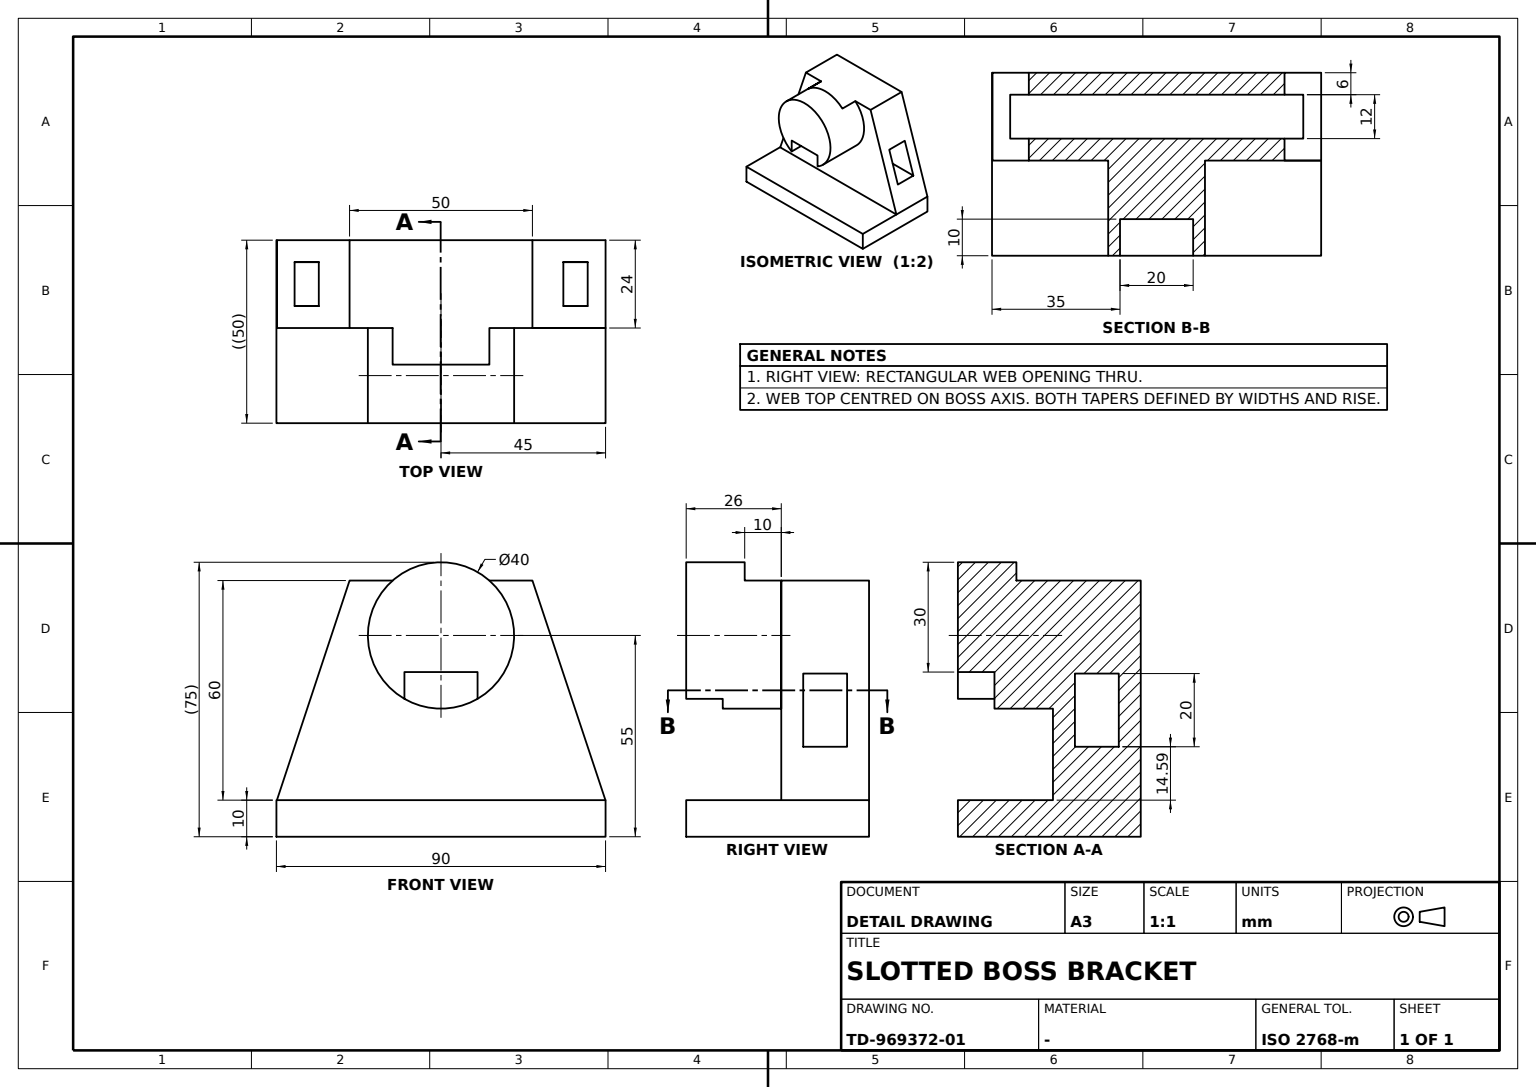
ISO-10303-21;
HEADER;
FILE_DESCRIPTION((''),'2;1');
FILE_NAME('','',(''),(''),'','','');
FILE_SCHEMA(('AUTOMOTIVE_DESIGN'));
ENDSEC;
DATA;
#1=APPLICATION_CONTEXT('');
#2=PRODUCT_CONTEXT('',#1,'mechanical');
#3=PRODUCT('','','',(#2));
#4=PRODUCT_DEFINITION_FORMATION('','',#3);
#5=PRODUCT_DEFINITION_CONTEXT('',#1,'design');
#6=PRODUCT_DEFINITION('','',#4,#5);
#7=PRODUCT_DEFINITION_SHAPE('','',#6);
#8=(LENGTH_UNIT()NAMED_UNIT(*)SI_UNIT(.MILLI.,.METRE.));
#9=(NAMED_UNIT(*)PLANE_ANGLE_UNIT()SI_UNIT($,.RADIAN.));
#10=(NAMED_UNIT(*)SI_UNIT($,.STERADIAN.)SOLID_ANGLE_UNIT());
#11=UNCERTAINTY_MEASURE_WITH_UNIT(LENGTH_MEASURE(0.005),#8,'distance_accuracy_value','');
#12=(GEOMETRIC_REPRESENTATION_CONTEXT(3)GLOBAL_UNCERTAINTY_ASSIGNED_CONTEXT((#11))GLOBAL_UNIT_ASSIGNED_CONTEXT((#8,#9,#10))REPRESENTATION_CONTEXT('',''));
#13=CARTESIAN_POINT('',(89.863327,0.,10.));
#14=VERTEX_POINT('',#13);
#15=CARTESIAN_POINT('',(90.,0.,10.));
#16=VERTEX_POINT('',#15);
#17=CARTESIAN_POINT('',(0.,0.,10.));
#18=DIRECTION('',(1.,0.,0.));
#19=VECTOR('',#18,1000.);
#20=LINE('',#17,#19);
#21=EDGE_CURVE('',#14,#16,#20,.T.);
#22=ORIENTED_EDGE('',*,*,#21,.F.);
#23=CARTESIAN_POINT('',(70.,0.,70.));
#24=VERTEX_POINT('',#23);
#25=CARTESIAN_POINT('',(89.898926,0.,9.892467));
#26=DIRECTION('',(-0.314280878,0.,0.949330043));
#27=VECTOR('',#26,1000.);
#28=LINE('',#25,#27);
#29=EDGE_CURVE('',#14,#24,#28,.T.);
#30=ORIENTED_EDGE('',*,*,#29,.T.);
#31=CARTESIAN_POINT('',(20.,0.,70.));
#32=VERTEX_POINT('',#31);
#33=LINE('',#31,#19);
#34=EDGE_CURVE('',#32,#24,#33,.T.);
#35=ORIENTED_EDGE('',*,*,#34,.F.);
#36=CARTESIAN_POINT('',(0.01789,0.,9.99951));
#37=VERTEX_POINT('',#36);
#38=DIRECTION('',(-0.315718471,0.,-0.948852911));
#39=VECTOR('',#38,1000.);
#40=LINE('',#31,#39);
#41=EDGE_CURVE('',#32,#37,#40,.T.);
#42=ORIENTED_EDGE('',*,*,#41,.T.);
#43=CARTESIAN_POINT('',(0.,0.,0.));
#44=VERTEX_POINT('',#43);
#45=DIRECTION('',(0.,0.,1.));
#46=VECTOR('',#45,1000.);
#47=LINE('',#43,#46);
#48=EDGE_CURVE('',#44,#37,#47,.T.);
#49=ORIENTED_EDGE('',*,*,#48,.F.);
#50=CARTESIAN_POINT('',(90.,0.,0.));
#51=VERTEX_POINT('',#50);
#52=LINE('',#43,#19);
#53=EDGE_CURVE('',#44,#51,#52,.T.);
#54=ORIENTED_EDGE('',*,*,#53,.T.);
#55=LINE('',#50,#46);
#56=EDGE_CURVE('',#51,#16,#55,.T.);
#57=ORIENTED_EDGE('',*,*,#56,.T.);
#58=EDGE_LOOP('',(#22,#30,#35,#42,#49,#54,#57));
#59=FACE_BOUND('',#58,.T.);
#60=DIRECTION('',(0.,-1.,0.));
#61=AXIS2_PLACEMENT_3D('',#43,#60,#18);
#62=PLANE('',#61);
#63=ADVANCED_FACE('',(#59),#62,.T.);
#64=ORIENTED_EDGE('',*,*,#56,.F.);
#65=CARTESIAN_POINT('',(90.,50.,0.));
#66=VERTEX_POINT('',#65);
#67=VECTOR('',#60,1000.);
#68=LINE('',#50,#67);
#69=EDGE_CURVE('',#66,#51,#68,.T.);
#70=ORIENTED_EDGE('',*,*,#69,.F.);
#71=CARTESIAN_POINT('',(90.,50.,10.));
#72=VERTEX_POINT('',#71);
#73=LINE('',#65,#46);
#74=EDGE_CURVE('',#66,#72,#73,.T.);
#75=ORIENTED_EDGE('',*,*,#74,.T.);
#76=LINE('',#15,#67);
#77=EDGE_CURVE('',#72,#16,#76,.T.);
#78=ORIENTED_EDGE('',*,*,#77,.T.);
#79=EDGE_LOOP('',(#64,#70,#75,#78));
#80=FACE_BOUND('',#79,.T.);
#81=DIRECTION('',(-1.,0.,0.));
#82=AXIS2_PLACEMENT_3D('',#65,#81,#60);
#83=PLANE('',#82);
#84=ADVANCED_FACE('',(#80),#83,.F.);
#85=CARTESIAN_POINT('',(20.,24.,70.));
#86=VERTEX_POINT('',#85);
#87=DIRECTION('',(0.,1.,0.));
#88=VECTOR('',#87,1000.);
#89=LINE('',#31,#88);
#90=EDGE_CURVE('',#32,#86,#89,.T.);
#91=ORIENTED_EDGE('',*,*,#90,.T.);
#92=CARTESIAN_POINT('',(0.01789,24.,10.));
#93=VERTEX_POINT('',#92);
#94=LINE('',#85,#39);
#95=EDGE_CURVE('',#86,#93,#94,.T.);
#96=ORIENTED_EDGE('',*,*,#95,.T.);
#97=CARTESIAN_POINT('',(0.,8.,10.));
#98=CARTESIAN_POINT('',(0.,16.,10.));
#99=CARTESIAN_POINT('',(0.,24.,10.));
#100=B_SPLINE_CURVE_WITH_KNOTS('',3,(#17,#97,#98,#99),.UNSPECIFIED.,.F.,.F.,(4,4),(0.00000025,23.999999778),.UNSPECIFIED.);
#101=EDGE_CURVE('',#37,#93,#100,.T.);
#102=ORIENTED_EDGE('',*,*,#101,.F.);
#103=ORIENTED_EDGE('',*,*,#41,.F.);
#104=EDGE_LOOP('',(#91,#96,#102,#103));
#105=FACE_BOUND('',#104,.T.);
#106=CARTESIAN_POINT('',(11.544207,6.,44.587158));
#107=VERTEX_POINT('',#106);
#108=CARTESIAN_POINT('',(4.889467,6.,24.587158));
#109=VERTEX_POINT('',#108);
#110=CARTESIAN_POINT('',(19.364536,6.,68.090191));
#111=LINE('',#110,#39);
#112=EDGE_CURVE('',#107,#109,#111,.T.);
#113=ORIENTED_EDGE('',*,*,#112,.T.);
#114=CARTESIAN_POINT('',(4.889467,18.,24.587158));
#115=VERTEX_POINT('',#114);
#116=LINE('',#114,#67);
#117=EDGE_CURVE('',#115,#109,#116,.T.);
#118=ORIENTED_EDGE('',*,*,#117,.F.);
#119=CARTESIAN_POINT('',(11.544207,18.,44.587158));
#120=VERTEX_POINT('',#119);
#121=CARTESIAN_POINT('',(13.373128,18.,50.083754));
#122=DIRECTION('',(0.315718471,0.,0.948852911));
#123=VECTOR('',#122,1000.);
#124=LINE('',#121,#123);
#125=EDGE_CURVE('',#115,#120,#124,.T.);
#126=ORIENTED_EDGE('',*,*,#125,.T.);
#127=LINE('',#106,#88);
#128=EDGE_CURVE('',#107,#120,#127,.T.);
#129=ORIENTED_EDGE('',*,*,#128,.F.);
#130=EDGE_LOOP('',(#113,#118,#126,#129));
#131=FACE_BOUND('',#130,.T.);
#132=DIRECTION('',(0.948852911,0.,-0.315718471));
#133=AXIS2_PLACEMENT_3D('',#31,#132,#38);
#134=PLANE('',#133);
#135=ADVANCED_FACE('',(#105,#131),#134,.F.);
#136=CARTESIAN_POINT('',(35.,40.,37.679492));
#137=VERTEX_POINT('',#136);
#138=CARTESIAN_POINT('',(35.,40.,45.));
#139=VERTEX_POINT('',#138);
#140=CARTESIAN_POINT('',(35.,40.,32.097708));
#141=LINE('',#140,#46);
#142=EDGE_CURVE('',#137,#139,#141,.T.);
#143=ORIENTED_EDGE('',*,*,#142,.T.);
#144=CARTESIAN_POINT('',(55.,40.,45.));
#145=VERTEX_POINT('',#144);
#146=VECTOR('',#81,1000.);
#147=LINE('',#144,#146);
#148=EDGE_CURVE('',#145,#139,#147,.T.);
#149=ORIENTED_EDGE('',*,*,#148,.F.);
#150=CARTESIAN_POINT('',(55.,40.,37.679492));
#151=VERTEX_POINT('',#150);
#152=DIRECTION('',(0.,0.,-1.));
#153=VECTOR('',#152,1000.);
#154=LINE('',#144,#153);
#155=EDGE_CURVE('',#145,#151,#154,.T.);
#156=ORIENTED_EDGE('',*,*,#155,.T.);
#157=CARTESIAN_POINT('',(45.,40.,55.));
#158=AXIS2_PLACEMENT_3D('',#157,#87,#45);
#159=CIRCLE('',#158,20.);
#160=EDGE_CURVE('',#151,#137,#159,.T.);
#161=ORIENTED_EDGE('',*,*,#160,.T.);
#162=EDGE_LOOP('',(#143,#149,#156,#161));
#163=FACE_BOUND('',#162,.T.);
#164=CARTESIAN_POINT('',(0.,40.,0.));
#165=AXIS2_PLACEMENT_3D('',#164,#87,#81);
#166=PLANE('',#165);
#167=ADVANCED_FACE('',(#163),#166,.T.);
#168=CARTESIAN_POINT('',(55.,50.,45.));
#169=VERTEX_POINT('',#168);
#170=CARTESIAN_POINT('',(55.,50.,37.679492));
#171=VERTEX_POINT('',#170);
#172=LINE('',#168,#153);
#173=EDGE_CURVE('',#169,#171,#172,.T.);
#174=ORIENTED_EDGE('',*,*,#173,.T.);
#175=LINE('',#170,#88);
#176=EDGE_CURVE('',#171,#151,#175,.F.);
#177=ORIENTED_EDGE('',*,*,#176,.T.);
#178=ORIENTED_EDGE('',*,*,#155,.F.);
#179=LINE('',#168,#67);
#180=EDGE_CURVE('',#169,#145,#179,.T.);
#181=ORIENTED_EDGE('',*,*,#180,.F.);
#182=EDGE_LOOP('',(#174,#177,#178,#181));
#183=FACE_BOUND('',#182,.T.);
#184=AXIS2_PLACEMENT_3D('',#168,#81,#152);
#185=PLANE('',#184);
#186=ADVANCED_FACE('',(#183),#185,.T.);
#187=ORIENTED_EDGE('',*,*,#29,.F.);
#188=CARTESIAN_POINT('',(89.863327,24.,10.));
#189=VERTEX_POINT('',#188);
#190=LINE('',#13,#88);
#191=EDGE_CURVE('',#14,#189,#190,.T.);
#192=ORIENTED_EDGE('',*,*,#191,.T.);
#193=CARTESIAN_POINT('',(70.,24.,70.));
#194=VERTEX_POINT('',#193);
#195=CARTESIAN_POINT('',(89.898926,24.,9.892467));
#196=LINE('',#195,#27);
#197=EDGE_CURVE('',#189,#194,#196,.T.);
#198=ORIENTED_EDGE('',*,*,#197,.T.);
#199=LINE('',#23,#88);
#200=EDGE_CURVE('',#24,#194,#199,.T.);
#201=ORIENTED_EDGE('',*,*,#200,.F.);
#202=EDGE_LOOP('',(#187,#192,#198,#201));
#203=FACE_BOUND('',#202,.T.);
#204=CARTESIAN_POINT('',(85.034168,18.,24.587158));
#205=VERTEX_POINT('',#204);
#206=CARTESIAN_POINT('',(78.41306,18.,44.587158));
#207=VERTEX_POINT('',#206);
#208=CARTESIAN_POINT('',(89.898926,18.,9.892467));
#209=LINE('',#208,#27);
#210=EDGE_CURVE('',#205,#207,#209,.T.);
#211=ORIENTED_EDGE('',*,*,#210,.F.);
#212=CARTESIAN_POINT('',(85.034168,6.,24.587158));
#213=VERTEX_POINT('',#212);
#214=CARTESIAN_POINT('',(85.034168,0.,24.587158));
#215=LINE('',#214,#67);
#216=EDGE_CURVE('',#205,#213,#215,.T.);
#217=ORIENTED_EDGE('',*,*,#216,.T.);
#218=CARTESIAN_POINT('',(78.41306,6.,44.587158));
#219=VERTEX_POINT('',#218);
#220=CARTESIAN_POINT('',(89.898926,6.,9.892467));
#221=DIRECTION('',(0.314280878,0.,-0.949330043));
#222=VECTOR('',#221,1000.);
#223=LINE('',#220,#222);
#224=EDGE_CURVE('',#219,#213,#223,.T.);
#225=ORIENTED_EDGE('',*,*,#224,.F.);
#226=CARTESIAN_POINT('',(78.41306,0.,44.587158));
#227=LINE('',#226,#88);
#228=EDGE_CURVE('',#219,#207,#227,.T.);
#229=ORIENTED_EDGE('',*,*,#228,.T.);
#230=EDGE_LOOP('',(#211,#217,#225,#229));
#231=FACE_BOUND('',#230,.T.);
#232=DIRECTION('',(-0.949330043,0.,-0.314280878));
#233=AXIS2_PLACEMENT_3D('',#25,#232,#26);
#234=PLANE('',#233);
#235=ADVANCED_FACE('',(#203,#231),#234,.F.);
#236=ORIENTED_EDGE('',*,*,#125,.F.);
#237=CARTESIAN_POINT('',(90.,18.,24.587158));
#238=LINE('',#237,#146);
#239=EDGE_CURVE('',#205,#115,#238,.T.);
#240=ORIENTED_EDGE('',*,*,#239,.F.);
#241=ORIENTED_EDGE('',*,*,#210,.T.);
#242=CARTESIAN_POINT('',(90.,18.,44.587158));
#243=LINE('',#242,#146);
#244=EDGE_CURVE('',#207,#120,#243,.T.);
#245=ORIENTED_EDGE('',*,*,#244,.T.);
#246=EDGE_LOOP('',(#236,#240,#241,#245));
#247=FACE_BOUND('',#246,.T.);
#248=AXIS2_PLACEMENT_3D('',#237,#60,#45);
#249=PLANE('',#248);
#250=ADVANCED_FACE('',(#247),#249,.T.);
#251=CARTESIAN_POINT('',(31.771243,34.,70.));
#252=VERTEX_POINT('',#251);
#253=CARTESIAN_POINT('',(31.771243,24.,70.));
#254=VERTEX_POINT('',#253);
#255=LINE('',#253,#88);
#256=EDGE_CURVE('',#252,#254,#255,.F.);
#257=ORIENTED_EDGE('',*,*,#256,.T.);
#258=LINE('',#85,#19);
#259=EDGE_CURVE('',#86,#254,#258,.T.);
#260=ORIENTED_EDGE('',*,*,#259,.F.);
#261=ORIENTED_EDGE('',*,*,#90,.F.);
#262=ORIENTED_EDGE('',*,*,#34,.T.);
#263=ORIENTED_EDGE('',*,*,#200,.T.);
#264=CARTESIAN_POINT('',(58.228757,24.,70.));
#265=VERTEX_POINT('',#264);
#266=EDGE_CURVE('',#265,#194,#258,.T.);
#267=ORIENTED_EDGE('',*,*,#266,.F.);
#268=CARTESIAN_POINT('',(58.228757,34.,70.));
#269=VERTEX_POINT('',#268);
#270=LINE('',#264,#88);
#271=EDGE_CURVE('',#265,#269,#270,.T.);
#272=ORIENTED_EDGE('',*,*,#271,.T.);
#273=CARTESIAN_POINT('',(0.,34.,70.));
#274=LINE('',#273,#146);
#275=EDGE_CURVE('',#269,#252,#274,.T.);
#276=ORIENTED_EDGE('',*,*,#275,.T.);
#277=EDGE_LOOP('',(#257,#260,#261,#262,#263,#267,#272,#276));
#278=FACE_BOUND('',#277,.T.);
#279=AXIS2_PLACEMENT_3D('',#31,#45,#18);
#280=PLANE('',#279);
#281=ADVANCED_FACE('',(#278),#280,.T.);
#282=CARTESIAN_POINT('',(35.,50.,37.679492));
#283=VERTEX_POINT('',#282);
#284=LINE('',#282,#88);
#285=EDGE_CURVE('',#283,#137,#284,.F.);
#286=ORIENTED_EDGE('',*,*,#285,.F.);
#287=CARTESIAN_POINT('',(35.,50.,45.));
#288=VERTEX_POINT('',#287);
#289=CARTESIAN_POINT('',(35.,50.,32.097708));
#290=LINE('',#289,#46);
#291=EDGE_CURVE('',#283,#288,#290,.T.);
#292=ORIENTED_EDGE('',*,*,#291,.T.);
#293=LINE('',#287,#67);
#294=EDGE_CURVE('',#288,#139,#293,.T.);
#295=ORIENTED_EDGE('',*,*,#294,.T.);
#296=ORIENTED_EDGE('',*,*,#142,.F.);
#297=EDGE_LOOP('',(#286,#292,#295,#296));
#298=FACE_BOUND('',#297,.T.);
#299=AXIS2_PLACEMENT_3D('',#289,#18,#45);
#300=PLANE('',#299);
#301=ADVANCED_FACE('',(#298),#300,.T.);
#302=ORIENTED_EDGE('',*,*,#74,.F.);
#303=CARTESIAN_POINT('',(0.,50.,0.));
#304=VERTEX_POINT('',#303);
#305=LINE('',#303,#146);
#306=EDGE_CURVE('',#66,#304,#305,.T.);
#307=ORIENTED_EDGE('',*,*,#306,.T.);
#308=CARTESIAN_POINT('',(0.,50.,10.));
#309=VERTEX_POINT('',#308);
#310=LINE('',#303,#46);
#311=EDGE_CURVE('',#304,#309,#310,.T.);
#312=ORIENTED_EDGE('',*,*,#311,.T.);
#313=LINE('',#308,#146);
#314=EDGE_CURVE('',#72,#309,#313,.T.);
#315=ORIENTED_EDGE('',*,*,#314,.F.);
#316=EDGE_LOOP('',(#302,#307,#312,#315));
#317=FACE_BOUND('',#316,.T.);
#318=AXIS2_PLACEMENT_3D('',#65,#87,#81);
#319=PLANE('',#318);
#320=ADVANCED_FACE('',(#317),#319,.T.);
#321=LINE('',#168,#146);
#322=EDGE_CURVE('',#169,#288,#321,.T.);
#323=ORIENTED_EDGE('',*,*,#322,.F.);
#324=ORIENTED_EDGE('',*,*,#180,.T.);
#325=ORIENTED_EDGE('',*,*,#148,.T.);
#326=ORIENTED_EDGE('',*,*,#294,.F.);
#327=EDGE_LOOP('',(#323,#324,#325,#326));
#328=FACE_BOUND('',#327,.T.);
#329=AXIS2_PLACEMENT_3D('',#168,#45,#81);
#330=PLANE('',#329);
#331=ADVANCED_FACE('',(#328),#330,.F.);
#332=ORIENTED_EDGE('',*,*,#173,.F.);
#333=ORIENTED_EDGE('',*,*,#322,.T.);
#334=ORIENTED_EDGE('',*,*,#291,.F.);
#335=CARTESIAN_POINT('',(45.,50.,55.));
#336=AXIS2_PLACEMENT_3D('',#335,#87,#45);
#337=CIRCLE('',#336,20.);
#338=EDGE_CURVE('',#283,#171,#337,.T.);
#339=ORIENTED_EDGE('',*,*,#338,.T.);
#340=EDGE_LOOP('',(#332,#333,#334,#339));
#341=FACE_BOUND('',#340,.T.);
#342=ADVANCED_FACE('',(#341),#319,.T.);
#343=ORIENTED_EDGE('',*,*,#239,.T.);
#344=ORIENTED_EDGE('',*,*,#117,.T.);
#345=CARTESIAN_POINT('',(90.,6.,24.587158));
#346=LINE('',#345,#146);
#347=EDGE_CURVE('',#213,#109,#346,.T.);
#348=ORIENTED_EDGE('',*,*,#347,.F.);
#349=ORIENTED_EDGE('',*,*,#216,.F.);
#350=EDGE_LOOP('',(#343,#344,#348,#349));
#351=FACE_BOUND('',#350,.T.);
#352=AXIS2_PLACEMENT_3D('',#237,#152,#60);
#353=PLANE('',#352);
#354=ADVANCED_FACE('',(#351),#353,.F.);
#355=ORIENTED_EDGE('',*,*,#53,.F.);
#356=LINE('',#43,#88);
#357=EDGE_CURVE('',#44,#304,#356,.T.);
#358=ORIENTED_EDGE('',*,*,#357,.T.);
#359=ORIENTED_EDGE('',*,*,#306,.F.);
#360=ORIENTED_EDGE('',*,*,#69,.T.);
#361=EDGE_LOOP('',(#355,#358,#359,#360));
#362=FACE_BOUND('',#361,.T.);
#363=AXIS2_PLACEMENT_3D('',#43,#45,#87);
#364=PLANE('',#363);
#365=ADVANCED_FACE('',(#362),#364,.F.);
#366=ORIENTED_EDGE('',*,*,#266,.T.);
#367=ORIENTED_EDGE('',*,*,#197,.F.);
#368=LINE('',#99,#19);
#369=EDGE_CURVE('',#93,#189,#368,.T.);
#370=ORIENTED_EDGE('',*,*,#369,.F.);
#371=ORIENTED_EDGE('',*,*,#95,.F.);
#372=ORIENTED_EDGE('',*,*,#259,.T.);
#373=CARTESIAN_POINT('',(45.,24.,55.));
#374=AXIS2_PLACEMENT_3D('',#373,#60,#152);
#375=CIRCLE('',#374,20.);
#376=EDGE_CURVE('',#265,#254,#375,.F.);
#377=ORIENTED_EDGE('',*,*,#376,.F.);
#378=EDGE_LOOP('',(#366,#367,#370,#371,#372,#377));
#379=FACE_BOUND('',#378,.T.);
#380=CARTESIAN_POINT('',(0.,24.,0.));
#381=AXIS2_PLACEMENT_3D('',#380,#60,#18);
#382=PLANE('',#381);
#383=ADVANCED_FACE('',(#379),#382,.F.);
#384=ORIENTED_EDGE('',*,*,#275,.F.);
#385=CARTESIAN_POINT('',(45.,34.,55.));
#386=AXIS2_PLACEMENT_3D('',#385,#60,#152);
#387=CIRCLE('',#386,20.);
#388=EDGE_CURVE('',#269,#252,#387,.T.);
#389=ORIENTED_EDGE('',*,*,#388,.T.);
#390=EDGE_LOOP('',(#384,#389));
#391=FACE_BOUND('',#390,.T.);
#392=CARTESIAN_POINT('',(0.,34.,0.));
#393=AXIS2_PLACEMENT_3D('',#392,#60,#18);
#394=PLANE('',#393);
#395=ADVANCED_FACE('',(#391),#394,.T.);
#396=ORIENTED_EDGE('',*,*,#314,.T.);
#397=LINE('',#17,#88);
#398=EDGE_CURVE('',#93,#309,#397,.T.);
#399=ORIENTED_EDGE('',*,*,#398,.F.);
#400=ORIENTED_EDGE('',*,*,#369,.T.);
#401=ORIENTED_EDGE('',*,*,#191,.F.);
#402=ORIENTED_EDGE('',*,*,#21,.T.);
#403=ORIENTED_EDGE('',*,*,#77,.F.);
#404=EDGE_LOOP('',(#396,#399,#400,#401,#402,#403));
#405=FACE_BOUND('',#404,.T.);
#406=AXIS2_PLACEMENT_3D('',#17,#45,#87);
#407=PLANE('',#406);
#408=ADVANCED_FACE('',(#405),#407,.T.);
#409=ORIENTED_EDGE('',*,*,#128,.T.);
#410=ORIENTED_EDGE('',*,*,#244,.F.);
#411=ORIENTED_EDGE('',*,*,#228,.F.);
#412=CARTESIAN_POINT('',(90.,6.,44.587158));
#413=LINE('',#412,#146);
#414=EDGE_CURVE('',#219,#107,#413,.T.);
#415=ORIENTED_EDGE('',*,*,#414,.T.);
#416=EDGE_LOOP('',(#409,#410,#411,#415));
#417=FACE_BOUND('',#416,.T.);
#418=AXIS2_PLACEMENT_3D('',#412,#45,#87);
#419=PLANE('',#418);
#420=ADVANCED_FACE('',(#417),#419,.F.);
#421=ORIENTED_EDGE('',*,*,#398,.T.);
#422=ORIENTED_EDGE('',*,*,#311,.F.);
#423=ORIENTED_EDGE('',*,*,#357,.F.);
#424=ORIENTED_EDGE('',*,*,#48,.T.);
#425=ORIENTED_EDGE('',*,*,#101,.T.);
#426=EDGE_LOOP('',(#421,#422,#423,#424,#425));
#427=FACE_BOUND('',#426,.T.);
#428=AXIS2_PLACEMENT_3D('',#43,#18,#87);
#429=PLANE('',#428);
#430=ADVANCED_FACE('',(#427),#429,.F.);
#431=ORIENTED_EDGE('',*,*,#160,.F.);
#432=ORIENTED_EDGE('',*,*,#176,.F.);
#433=ORIENTED_EDGE('',*,*,#338,.F.);
#434=ORIENTED_EDGE('',*,*,#285,.T.);
#435=EDGE_LOOP('',(#431,#432,#433,#434));
#436=FACE_BOUND('',#435,.T.);
#437=ORIENTED_EDGE('',*,*,#388,.F.);
#438=ORIENTED_EDGE('',*,*,#271,.F.);
#439=ORIENTED_EDGE('',*,*,#376,.T.);
#440=ORIENTED_EDGE('',*,*,#256,.F.);
#441=EDGE_LOOP('',(#437,#438,#439,#440));
#442=FACE_BOUND('',#441,.T.);
#443=CARTESIAN_POINT('',(45.,37.,55.));
#444=AXIS2_PLACEMENT_3D('',#443,#87,#81);
#445=CYLINDRICAL_SURFACE('',#444,20.);
#446=ADVANCED_FACE('',(#436,#442),#445,.T.);
#447=ORIENTED_EDGE('',*,*,#112,.F.);
#448=ORIENTED_EDGE('',*,*,#414,.F.);
#449=ORIENTED_EDGE('',*,*,#224,.T.);
#450=ORIENTED_EDGE('',*,*,#347,.T.);
#451=EDGE_LOOP('',(#447,#448,#449,#450));
#452=FACE_BOUND('',#451,.T.);
#453=AXIS2_PLACEMENT_3D('',#412,#87,#152);
#454=PLANE('',#453);
#455=ADVANCED_FACE('',(#452),#454,.T.);
#456=CLOSED_SHELL('',(#63,#84,#135,#167,#186,#235,#250,#281,#301,#320,#331,#342,#354,#365,#383,#395,#408,#420,#430,#446,#455));
#457=MANIFOLD_SOLID_BREP('',#456);
#458=ADVANCED_BREP_SHAPE_REPRESENTATION('',(#457),#12);
#459=SHAPE_DEFINITION_REPRESENTATION(#7,#458);
ENDSEC;
END-ISO-10303-21;
